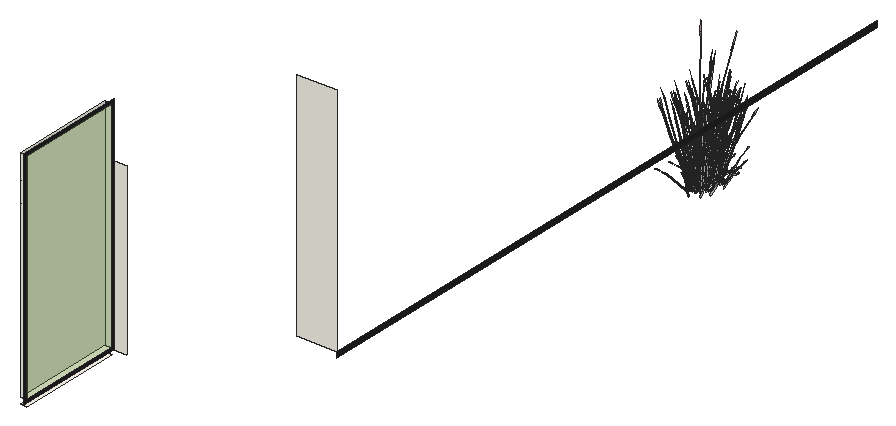
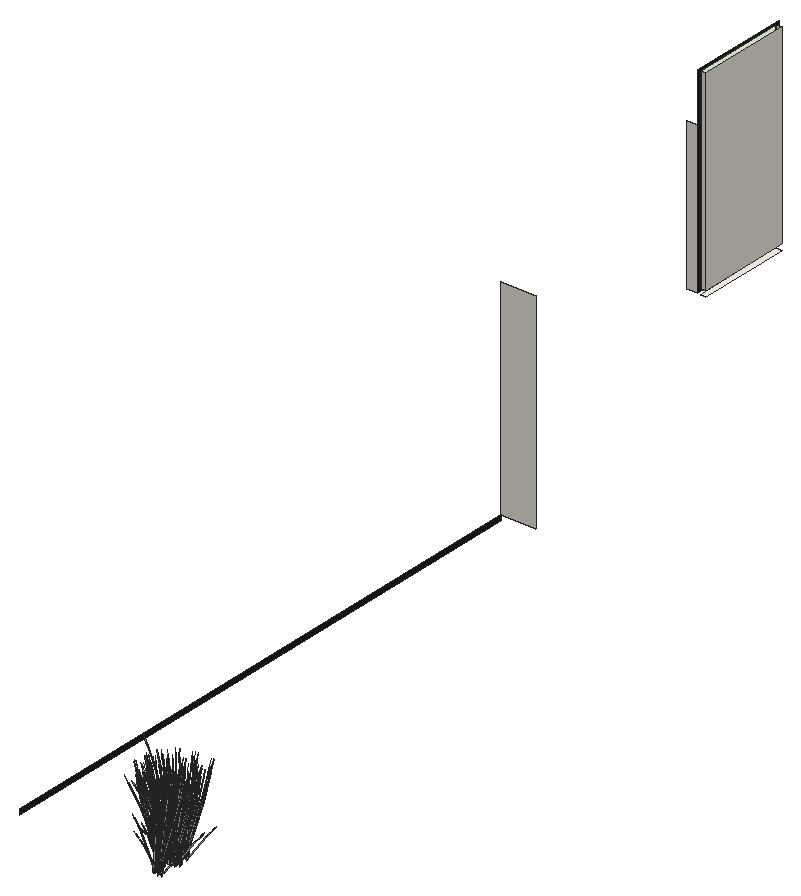
# SketchUp Ruby script. Lengths in inches.
U = 1.inch
M = Sketchup.active_model
def pt(a) = Geom::Point3d.new(a.map { |v| v * U })
def face(e, loops, mat)
  f = e.add_face(loops[0].map { |a| pt(a) })
  loops[1..].each { |l| e.add_face(l.map { |a| pt(a) }).erase! }
  f.material = f.back_material = mat if mat
  f
end
# faces: each face lists its corners as indices into pts; further lists are holes
def faces(e, pts, list, mat = nil) = list.each { |f| face(e, (f[0].is_a?(Array) ? f : [f]).map { |l| l.map { |i| pts[i] } }, mat) }
# xy, xz, yz: faces in a plane at the given z, y or x. An outline is a flat list of corners, or four numbers for a rectangle; further outlines are holes
def ring(l) = l.size == 4 ? [[l[0], l[1]], [l[2], l[1]], [l[2], l[3]], [l[0], l[3]]] : l.each_slice(2).to_a
def flat(e, list, mat, &to3) = list.each { |f| face(e, (f[0].is_a?(Array) ? f : [f]).map { |l| ring(l).map { |u, v| to3.(u, v) } }, mat) }
def xy(e, z, list, mat = nil) = flat(e, list, mat) { |x, y| [x, y, z] }
def xz(e, y, list, mat = nil) = flat(e, list, mat) { |x, z| [x, y, z] }
def yz(e, x, list, mat = nil) = flat(e, list, mat) { |y, z| [x, y, z] }
def lines(e, pts, list) = list.each { |a, b| e.add_line(pt(pts[a]), pt(pts[b])) }
# prism: a flat outline (further loops are holes) pulled along v
def prism(e, loops, v, mat = nil)
  f = face(e, loops, mat); d = Geom::Vector3d.new(v.map { |x| x * U })
  f.pushpull(f.normal.samedirection?(d) ? d.length : -d.length)
end
def box(e, o, s, mat = nil) = prism(e, [[o, [o[0] + s[0], o[1], o[2]], [o[0] + s[0], o[1] + s[1], o[2]], [o[0], o[1] + s[1], o[2]]]], [0, 0, s[2]], mat)
def at(x, y, z, deg = 0) = Geom::Transformation.translation(pt([x, y, z])) * Geom::Transformation.rotation(ORIGIN, Z_AXIS, deg.degrees)
def axes(o, x, y, z) = Geom::Transformation.new([*x, 0, *y, 0, *z, 0, *pt(o).to_a, 1])
def part(name) = M.definitions.add(name)
# library, detail: a bought-in or finely detailed component or shape, given as its bounding box
def library(name, o, s) = part(name).tap { |d| box(d.entities, o, s) }
def detail(e, o, s) = box(e.add_group.entities, o, s)
def put(e, d, t, mat = nil) = e.add_instance(d, t).tap { |i| i.material = mat if mat }
def group(e, t, mat = nil) = e.add_group.tap { |g| g.transformation = t; g.material = mat if mat }.entities
root = M.entities
M.materials.add("C01_Vanilla_Cream").color = [255, 251, 241]
M.materials.add("Glass_Basic_01").color = [119, 186, 61]
M.materials["Glass_Basic_01"].alpha = 0.25
M.materials.add("LightPink_Translucent").color = [144, 107, 117]
M.materials["LightPink_Translucent"].alpha = 0.75
M.materials.add("Marble_07_1K").color = [36, 34, 36]
c1 = part("blade")
p = [[2.15,0.21,22],[0,0.17,0],[0.09,0.45,0],[2.18,0.31,22],[2.29,0.31,22],[0.38,0.45,0],
  [2.48,0.24,33],[2.49,0.24,33],[2.48,0.22,33]]
faces(c1.entities,p,[[0,1,2,3],[4,5,2,3],[6,3,4,7],[8,0,3,6]])
c2 = part("seeds")
p = [[0.3,-0.1,1.38],[-0.01,-0.03,1.59],[-0.01,-0.03,0.03],[0.14,-0.07,-0.07],[0.29,-0.03,3],[0.15,0.01,3.11]]
faces(c2.entities,p,[[0,1,2,3],[1,0,4,5]],"LightPink_Translucent")
c3 = part("blade with seeds")
put(c3.entities,c1,at(0,0,0))
put(c3.entities,c2,axes([2.4,0.25,30.99],[1.5799,-0.05474,1.17369],[-0.12525,1.92788,0.29478],[-0.07173,-0.02425,1.56792]))
xy(root,335,[[700,25,702,59]],"C01_Vanilla_Cream")
xy(root,337,[[700,25,702,59]],"C01_Vanilla_Cream")
xz(root,25,[[700,337,702,407]],"C01_Vanilla_Cream")
xz(root,59,[[700,337,702,407]],"C01_Vanilla_Cream")
xz(root,60,[[702,336,706,390]],"C01_Vanilla_Cream")
xz(root,144,[[693.41,300,706,375]],"C01_Vanilla_Cream")
yz(root,700,[[25,337,59,407]],"C01_Vanilla_Cream")
yz(root,702,[[25,337,59,407]],"Glass_Basic_01")
yz(root,702,[[[24,336,60,408],[25,337,59,407]]],"Marble_07_1K")
yz(root,706,[[144,298,360,300]],"Marble_07_1K")
put(root,c3,axes([687.37,307.125,267.91],[-0.09951,-0.08005,1.45204],[-0.66407,0.05075,-0.22964],[-0.10598,-0.19148,0.11645]))
put(root,c3,axes([688.0625,308.48,268.13],[-0.31051,-0.46426,-0.58968],[0.63919,-0.25873,0.07116],[-0.07261,-0.22432,0.83415]))
put(root,c3,axes([689.35,308.93,268.13],[0.01693,-0.52814,-0.58968],[0.71285,0.03547,0.07116],[0.07523,-0.22375,0.83415]))
put(root,c3,axes([690.35,308.11,267.91],[-0.00628,-0.11364,1.45204],[-0.53042,-0.32843,-0.22964],[0.08201,-0.19909,0.11645]))
put(root,c3,axes([688.12,308.08,267.76],[0.19614,-0.43908,-0.29394],[0.57222,0.12807,0.37948],[-0.05247,-0.17678,0.72609]))
put(root,c3,axes([688.55,308.66,267.22],[-0.12114,0.19625,1.42242],[-0.50818,-0.40613,0.11501],[0.22925,-0.25313,0.60807]))
put(root,c3,axes([690.21,307.7,267.91],[-0.06607,0.04361,1.47228],[-0.64734,-0.14714,-0.13912],[-0.02343,-0.19032,0.26054]))
put(root,c3,axes([687.83,308.38,267.89],[-0.63954,-0.14313,-0.42412],[0.21921,-0.49074,-0.32852],[-0.05864,-0.19758,0.81151]))
put(root,c3,axes([688.22,307.16,266.3],[0.08346,0.33295,0.95334],[-0.46298,-0.1844,0.70045],[0.04982,-0.17048,0.20998]))
put(root,c3,axes([689.21,308.76,267.89],[-0.46573,-0.38364,-0.42412],[0.49199,-0.33598,-0.32852],[0.07086,-0.19492,0.81151]))
put(root,c3,axes([688.19,308.18,267.93],[0.64106,0.14927,0.39842],[-0.21921,0.49074,0.32852],[-0.03852,-0.19299,0.82444]))
put(root,c3,axes([688.375,308.36,268.18],[-0.63664,0.26583,-0.10093],[-0.31286,-0.47181,-0.56021],[-0.084,-0.19882,0.85122]))
put(root,c3,axes([689.7,308.96,268.18],[-0.71502,-0.02829,-0.10093],[0.01954,-0.53563,-0.56021],[0.04967,-0.20629,0.85122]))
put(root,c3,axes([689.65,308.61,267.76],[0.4402,-0.30062,-0.29394],[0.41671,0.34326,0.37948],[0.0634,-0.1744,0.72609]))
put(root,c3,axes([688.36,308.15,267.93],[0.47939,-0.19405,0.05337],[0.23464,0.35385,0.42015],[-0.0463,-0.15598,0.64067]))
put(root,c3,axes([688.18,308.55,268.19],[-0.19614,0.43908,0.29394],[-0.57222,-0.12807,-0.37948],[-0.05247,-0.17678,0.72609]))
put(root,c3,axes([689.65,308.73,267.93],[0.46327,0.38957,0.39842],[-0.49199,0.33598,0.32852],[0.08546,-0.18277,0.82444]))
put(root,c3,axes([689.82,308.77,267.93],[0.53464,0.0266,0.05337],[-0.01466,0.40172,0.42015],[0.05594,-0.15388,0.64067]))
put(root,c3,axes([689.42,309.04,268.19],[-0.4402,0.30062,0.29394],[-0.41671,-0.34326,-0.37948],[0.0634,-0.1744,0.72609]))
put(root,c3,axes([690.19,309.85,268.13],[0.33983,-0.45051,-0.58968],[0.59551,0.32017,0.07116],[0.20291,-0.16322,0.83415]))
put(root,c3,axes([690.18,309.64,267.89],[-0.16713,-0.52135,-0.42412],[0.63294,-0.0912,-0.32852],[0.18138,-0.14003,0.81151]))
put(root,c3,axes([690.48,310.01,268.18],[-0.60181,-0.31483,-0.10093],[0.34671,-0.45593,-0.56021],[0.17003,-0.15849,0.85122]))
put(root,c3,axes([691.96,309.875,267.91],[-0.08498,-0.00434,1.47228],[-0.35287,-0.46464,-0.13912],[0.14171,-0.15278,0.26054]))
put(root,c3,axes([690.95,308.6,266.3],[-0.2167,0.29065,0.95334],[-0.18626,-0.3905,0.70045],[0.17898,-0.09785,0.20998]))
put(root,c3,axes([690.64,309.69,267.76],[0.56631,-0.0816,-0.29394],[0.14954,0.46647,0.37948],[0.16229,-0.12529,0.72609]))
put(root,c3,axes([690.18,309.97,268.19],[-0.56631,0.0816,0.29394],[-0.14954,-0.46647,-0.37948],[0.16229,-0.12529,0.72609]))
put(root,c3,axes([690.7,309.9,267.93],[0.44663,0.24013,0.05337],[-0.26003,0.34195,0.42015],[0.14319,-0.11055,0.64067]))
put(root,c3,axes([690.57,309.79,267.93],[0.16135,0.52549,0.39842],[-0.63294,0.0912,0.32852],[0.18654,-0.12359,0.82444]))
put(root,c3,axes([692.28,310.43,267.91],[0.09028,-0.08697,1.45204],[-0.11555,-0.53348,-0.22964],[0.22652,-0.10115,0.11645]))
put(root,c3,axes([687.79,312.07,267.91],[-0.09951,-0.08005,1.45204],[-0.66407,0.05075,-0.22964],[-0.10598,-0.19148,0.11645]))
put(root,c3,axes([688.48,313.42,268.13],[-0.31051,-0.46426,-0.58968],[0.63919,-0.25873,0.07116],[-0.07261,-0.22432,0.83415]))
put(root,c3,axes([689.78,313.875,268.13],[0.01693,-0.52814,-0.58968],[0.71285,0.03547,0.07116],[0.07523,-0.22375,0.83415]))
put(root,c3,axes([690.5,311.24,268.18],[-0.32734,-0.51701,-0.10093],[0.58097,-0.25407,-0.56021],[0.24483,-0.06821,0.85122]))
put(root,c3,axes([690.77,313.05,267.91],[-0.00628,-0.11364,1.45204],[-0.53042,-0.32843,-0.22964],[0.08201,-0.19909,0.11645]))
put(root,c3,axes([688.54,313.03,267.76],[0.19614,-0.43908,-0.29394],[0.57222,0.12807,0.37948],[-0.05247,-0.17678,0.72609]))
put(root,c3,axes([690.47,310.8,267.89],[0.17625,-0.51936,-0.42412],[0.60429,0.17802,-0.32852],[0.2433,-0.04762,0.81151]))
put(root,c3,axes([688.98,313.61,267.22],[-0.12114,0.19625,1.42242],[-0.50818,-0.40613,0.11501],[0.22925,-0.25313,0.60807]))
put(root,c3,axes([690.63,312.64,267.91],[-0.06607,0.04361,1.47228],[-0.64734,-0.14714,-0.13912],[-0.02343,-0.19032,0.26054]))
put(root,c3,axes([688.25,313.33,267.89],[-0.63954,-0.14313,-0.42412],[0.21921,-0.49074,-0.32852],[-0.05864,-0.19758,0.81151]))
put(root,c3,axes([688.65,312.1,266.3],[0.08346,0.33295,0.95334],[-0.46298,-0.1844,0.70045],[0.04982,-0.17048,0.20998]))
put(root,c3,axes([689.63,313.7,267.89],[-0.46573,-0.38364,-0.42412],[0.49199,-0.33598,-0.32852],[0.07086,-0.19492,0.81151]))
put(root,c3,axes([690.36,310.99,268.13],[0.57168,-0.25217,-0.58968],[0.3186,0.51908,0.07116],[0.27622,-0.05897,0.83415]))
put(root,c3,axes([688.61,313.13,267.93],[0.64106,0.14927,0.39842],[-0.21921,0.49074,0.32852],[-0.03852,-0.19299,0.82444]))
put(root,c3,axes([690.27,311.08,268.19],[-0.54068,-0.15928,0.29394],[0.1577,-0.46469,-0.37948],[0.21769,-0.04261,0.72609]))
put(root,c3,axes([688.8,313.3,268.18],[-0.63664,0.26583,-0.10093],[-0.31286,-0.47181,-0.56021],[-0.084,-0.19882,0.85122]))
put(root,c3,axes([690.12,313.9,268.18],[-0.71502,-0.02829,-0.10093],[0.01954,-0.53563,-0.56021],[0.04967,-0.20629,0.85122]))
put(root,c3,axes([690.07,313.56,267.76],[0.4402,-0.30062,-0.29394],[0.41671,0.34326,0.37948],[0.0634,-0.1744,0.72609]))
put(root,c3,axes([688.78,313.09,267.93],[0.47939,-0.19405,0.05337],[0.23464,0.35385,0.42015],[-0.0463,-0.15598,0.64067]))
put(root,c3,axes([687.14,313.14,267.93],[0.29569,-0.36271,0.05337],[0.42107,0.21117,0.42015],[-0.13613,-0.11629,0.64067]))
put(root,c3,axes([690.84,311.03,267.76],[0.54068,0.15928,-0.29394],[-0.1577,0.46469,0.37948],[0.21769,-0.04261,0.72609]))
put(root,c3,axes([688.61,313.49,268.19],[-0.19614,0.43908,0.29394],[-0.57222,-0.12807,-0.37948],[-0.05247,-0.17678,0.72609]))
put(root,c3,axes([689.37,310.46,267.22],[-0.26985,0.01293,1.42242],[0.17902,-0.56047,0.11501],[0.38456,0.03467,0.60807]))
put(root,c3,axes([690.07,313.67,267.93],[0.46327,0.38957,0.39842],[-0.49199,0.33598,0.32852],[0.08546,-0.18277,0.82444]))
put(root,c3,axes([690.24,313.71,267.93],[0.53464,0.0266,0.05337],[-0.01466,0.40172,0.42015],[0.05594,-0.15388,0.64067]))
put(root,c3,axes([690.76,311.23,267.93],[0.23895,0.38931,0.05337],[-0.43573,0.19055,0.42015],[0.19208,-0.0376,0.64067]))
put(root,c3,axes([689.84,313.98,268.19],[-0.4402,0.30062,0.29394],[-0.41671,-0.34326,-0.37948],[0.0634,-0.1744,0.72609]))
put(root,c3,axes([690.72,311.09,267.93],[-0.18381,0.5206,0.39842],[-0.60429,-0.17802,0.32852],[0.23764,-0.03129,0.82444]))
put(root,c3,axes([690.62,314.79,268.13],[0.33983,-0.45051,-0.58968],[0.59551,0.32017,0.07116],[0.20291,-0.16322,0.83415]))
put(root,c3,axes([690.6,314.58,267.89],[-0.16713,-0.52135,-0.42412],[0.63294,-0.0912,-0.32852],[0.18138,-0.14003,0.81151]))
put(root,c3,axes([690.9,314.95,268.18],[-0.60181,-0.31483,-0.10093],[0.34671,-0.45593,-0.56021],[0.17003,-0.15849,0.85122]))
put(root,c3,axes([691.99,311.13,266.3],[-0.40197,0.09426,0.95334],[0.18921,-0.38956,0.70045],[0.21325,0.02666,0.20998]))
put(root,c3,axes([692.38,314.82,267.91],[-0.08498,-0.00434,1.47228],[-0.35287,-0.46464,-0.13912],[0.14171,-0.15278,0.26054]))
put(root,c3,axes([691.8,312.78,267.91],[-0.05883,-0.04999,1.47228],[0.12868,-0.53581,-0.13912],[0.23172,-0.03423,0.26054]))
put(root,c3,axes([691.38,313.54,266.3],[-0.2167,0.29065,0.95334],[-0.18626,-0.3905,0.70045],[0.17898,-0.09785,0.20998]))
put(root,c3,axes([691.29,312.33,267.26],[-0.12452,-0.47997,-0.02898],[0.58854,-0.11034,-0.1314],[0.1229,0.03043,0.43341]))
put(root,c3,axes([689.77,312.31,268.18],[0.03484,-0.58066,-0.10093],[0.65957,0.01587,-0.56021],[0.25402,0.04034,0.85122]))
put(root,c3,axes([691.07,314.64,267.76],[0.56631,-0.0816,-0.29394],[0.14954,0.46647,0.37948],[0.16229,-0.12529,0.72609]))
put(root,c3,axes([689.66,312.09,268.19],[-0.37017,-0.35748,0.29394],[0.42268,-0.3384,-0.37948],[0.21476,0.05149,0.72609]))
put(root,c3,axes([690.61,314.91,268.19],[-0.56631,0.0816,0.29394],[-0.14954,-0.46647,-0.37948],[0.16229,-0.12529,0.72609]))
put(root,c3,axes([690.34,311.97,267.91],[0.13956,-0.00966,1.45204],[0.38281,-0.44358,-0.22964],[0.24825,0.05855,0.11645]))
put(root,c3,axes([691.12,314.84,267.93],[0.44663,0.24013,0.05337],[-0.26003,0.34195,0.42015],[0.14319,-0.11055,0.64067]))
put(root,c3,axes([690.99,314.74,267.93],[0.16135,0.52549,0.39842],[-0.63294,0.0912,0.32852],[0.18654,-0.12359,0.82444]))
put(root,c3,axes([689.8,312.04,268.13],[0.65035,0.01375,-0.58968],[-0.04368,0.5789,0.07116],[0.27552,0.06109,0.83415]))
put(root,c3,axes([692.7,315.37,267.91],[0.09028,-0.08697,1.45204],[-0.11555,-0.53348,-0.22964],[0.22652,-0.10115,0.11645]))
put(root,c3,axes([690.1875,312.27,267.76],[0.37017,0.35748,-0.29394],[-0.42268,0.3384,0.37948],[0.21476,0.05149,0.72609]))
put(root,c3,axes([690,312.41,267.93],[-0.03276,0.43418,0.05337],[-0.49468,-0.0119,0.42015],[0.18949,0.04543,0.64067]))
put(root,c3,axes([690.04,312.27,267.93],[-0.47971,0.37622,0.39842],[-0.41372,-0.39954,0.32852],[0.22506,0.0694,0.82444]))
put(root,c3,axes([690.92,316.18,268.18],[-0.32734,-0.51701,-0.10093],[0.58097,-0.25407,-0.56021],[0.24483,-0.06821,0.85122]))
put(root,c3,axes([690.89,315.74,267.89],[0.17625,-0.51936,-0.42412],[0.60429,0.17802,-0.32852],[0.2433,-0.04762,0.81151]))
put(root,c3,axes([688.52,312.71,268.19],[-0.10048,-0.4599,0.29394],[0.5744,-0.12144,-0.37948],[0.15428,0.13179,0.72609]))
put(root,c3,axes([688.86,311.36,267.22],[-0.24166,-0.09837,1.42242],[0.50011,-0.41269,0.11501],[0.3117,0.18617,0.60807]))
put(root,c3,axes([688.91,310.0625,267.71],[-0.56218,-0.29666,1.14775],[0.59361,-0.46189,0.49522],[0.18138,0.27836,1.10941]))
put(root,c3,axes([690.78,315.93,268.13],[0.57168,-0.25217,-0.58968],[0.3186,0.51908,0.07116],[0.27622,-0.05897,0.83415]))
put(root,c3,axes([689.75,312.48,266.3],[-0.36631,-0.16417,0.95334],[0.47299,-0.16681,0.70045],[0.12758,0.1413,0.20998]))
put(root,c3,axes([688.47,312.95,268.18],[0.38768,-0.48872,-0.10093],[0.56143,0.28156,-0.56021],[0.19516,0.13808,0.85122]))
put(root,c3,axes([690.7,316.03,268.19],[-0.54068,-0.15928,0.29394],[0.1577,-0.46469,-0.37948],[0.21769,-0.04261,0.72609]))
put(root,c3,axes([687.33,318.61,267.91],[-0.09951,-0.08005,1.45204],[-0.66407,0.05075,-0.22964],[-0.10598,-0.19148,0.11645]))
put(root,c3,axes([685.91,312.29,268.19],[0.4402,-0.30062,0.29394],[0.41671,0.34326,-0.37948],[-0.0634,0.1744,0.72609]))
put(root,c3,axes([687.96,313.35,267.91],[0.00193,-0.06913,1.47228],[0.55753,-0.30498,-0.13912],[0.19366,0.10886,0.26054]))
put(root,c3,axes([688.03,319.96,268.13],[-0.31051,-0.46426,-0.58968],[0.63919,-0.25873,0.07116],[-0.07261,-0.22432,0.83415]))
put(root,c3,axes([688.86,310.63,266.36],[-0.01777,-0.53759,1.17256],[0.80434,0.13935,0.49647],[-0.19024,0.29416,1.1068]))
put(root,c3,axes([688.93,312.7,267.89],[0.64198,-0.13573,-0.42412],[0.1123,0.514,-0.32852],[0.17243,0.1473,0.81151]))
put(root,c3,axes([687.15,312.78,268.19],[0.19614,-0.43908,0.29394],[0.57222,0.12807,-0.37948],[0.05247,0.17678,0.72609]))
put(root,c3,axes([691.27,315.98,267.76],[0.54068,0.15928,-0.29394],[-0.1577,0.46469,0.37948],[0.21769,-0.04261,0.72609]))
put(root,c3,axes([689.32,320.41,268.13],[0.01693,-0.52814,-0.58968],[0.71285,0.03547,0.07116],[0.07523,-0.22375,0.83415]))
put(root,c3,axes([688.61,313.125,267.93],[-0.29569,0.36271,0.05337],[-0.42107,-0.21117,0.42015],[0.13613,0.11629,0.64067]))
put(root,c3,axes([690.3125,319.59,267.91],[-0.00628,-0.11364,1.45204],[-0.53042,-0.32843,-0.22964],[0.08201,-0.19909,0.11645]))
put(root,c3,axes([688.09,319.57,267.76],[0.19614,-0.43908,-0.29394],[0.57222,0.12807,0.37948],[-0.05247,-0.17678,0.72609]))
put(root,c3,axes([688.52,320.15,267.22],[-0.12114,0.19625,1.42242],[-0.50818,-0.40613,0.11501],[0.22925,-0.25313,0.60807]))
put(root,c3,axes([690.17,319.18,267.91],[-0.06607,0.04361,1.47228],[-0.64734,-0.14714,-0.13912],[-0.02343,-0.19032,0.26054]))
put(root,c3,axes([687.92,314.35,268.6875],[0.44958,-0.32756,-0.05385],[0.41194,0.35875,-0.24415],[0.029,0.10165,0.8053]))
put(root,c3,axes([688.73,313.02,267.93],[-0.64708,0.13103,0.39842],[-0.1123,-0.514,0.32852],[0.15218,0.15149,0.82444]))
put(root,c3,axes([689.79,315.4,267.22],[-0.26985,0.01293,1.42242],[0.17902,-0.56047,0.11501],[0.38456,0.03467,0.60807]))
put(root,c3,axes([687.79,319.87,267.89],[-0.63954,-0.14313,-0.42412],[0.21921,-0.49074,-0.32852],[-0.05864,-0.19758,0.81151]))
put(root,c3,axes([688.19,318.64,266.3],[0.08346,0.33295,0.95334],[-0.46298,-0.1844,0.70045],[0.04982,-0.17048,0.20998]))
put(root,c3,axes([689.18,320.24,267.89],[-0.46573,-0.38364,-0.42412],[0.49199,-0.33598,-0.32852],[0.07086,-0.19492,0.81151]))
put(root,c3,axes([691.19,316.17,267.93],[0.23895,0.38931,0.05337],[-0.43573,0.19055,0.42015],[0.19208,-0.0376,0.64067]))
put(root,c3,axes([691.14,316.03,267.93],[-0.18381,0.5206,0.39842],[-0.60429,-0.17802,0.32852],[0.23764,-0.03129,0.82444]))
put(root,c3,axes([686.97,313.18,267.93],[-0.47939,0.19405,0.05337],[-0.23464,-0.35385,0.42015],[0.0463,0.15598,0.64067]))
put(root,c3,axes([685.63,312.37,268.48],[0.71502,0.02829,-0.11203],[-0.01954,0.53563,-0.62183],[-0.04967,0.20629,0.94486]))
put(root,c3,axes([686.95,312.97,268.18],[0.63664,-0.26583,-0.10093],[0.31286,0.47181,-0.56021],[0.084,0.19882,0.85122]))
put(root,c3,axes([687.14,313.14,268.2],[-0.64106,-0.14927,0.44225],[0.21921,-0.49074,0.36465],[0.03852,0.19299,0.91512]))
put(root,c3,axes([688.16,319.67,267.93],[0.64106,0.14927,0.39842],[-0.21921,0.49074,0.32852],[-0.03852,-0.19299,0.82444]))
put(root,c3,axes([688.34,319.84,268.18],[-0.63664,0.26583,-0.10093],[-0.31286,-0.47181,-0.56021],[-0.084,-0.19882,0.85122]))
put(root,c3,axes([689.66,320.44,268.18],[-0.71502,-0.02829,-0.10093],[0.01954,-0.53563,-0.56021],[0.04967,-0.20629,0.85122]))
put(root,c3,axes([689.61,320.1,267.76],[0.4402,-0.30062,-0.29394],[0.41671,0.34326,0.37948],[0.0634,-0.1744,0.72609]))
put(root,c3,axes([688.33,319.63,267.93],[0.47939,-0.19405,0.05337],[0.23464,0.35385,0.42015],[-0.0463,-0.15598,0.64067]))
put(root,c3,axes([692.41,316.07,266.3],[-0.40197,0.09426,0.95334],[0.18921,-0.38956,0.70045],[0.21325,0.02666,0.20998]))
put(root,c3,axes([686.12,312.57,268.15],[0.46573,0.38364,-0.47077],[-0.49199,0.33598,-0.36465],[-0.07086,0.19492,0.90078]))
put(root,c3,axes([687.5,312.94,267.89],[0.63954,0.14313,-0.42412],[-0.21921,0.49074,-0.32852],[0.05864,0.19758,0.81151]))
put(root,c3,axes([687.86,311.93,267.22],[-0.14872,-0.18332,1.42242],[0.6872,-0.15433,0.11501],[0.15531,0.28779,0.60807]))
put(root,c3,axes([692.23,317.72,267.91],[-0.05883,-0.04999,1.47228],[0.12868,-0.53581,-0.13912],[0.23172,-0.03423,0.26054]))
put(root,c3,axes([687.21,313.24,267.76],[-0.19614,0.43908,-0.29394],[-0.57222,-0.12807,0.37948],[0.05247,0.17678,0.72609]))
